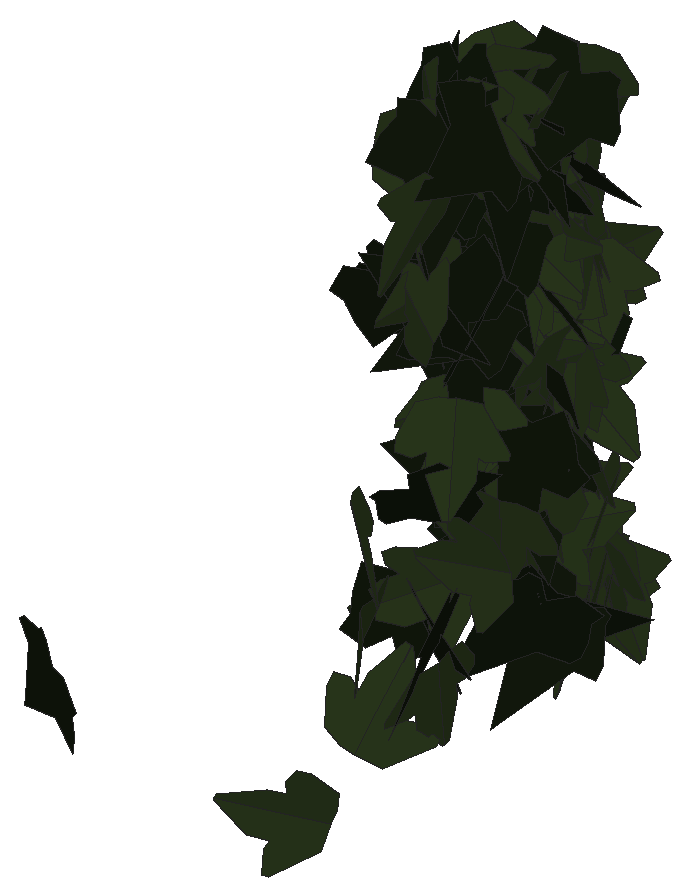
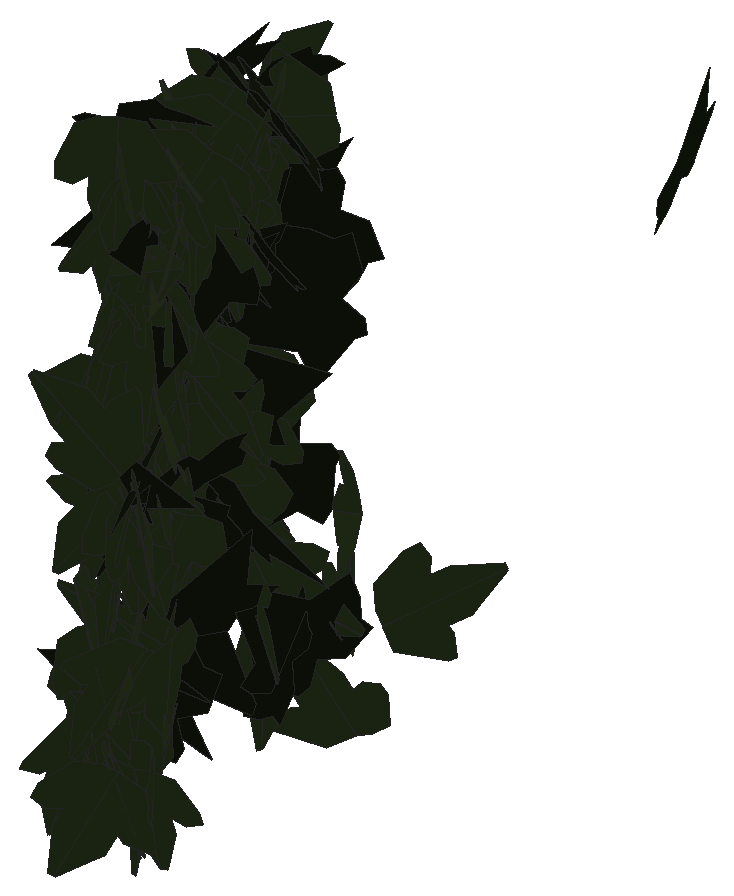
# SketchUp Ruby script. Lengths in inches.
U = 1.inch
M = Sketchup.active_model
def pt(a) = Geom::Point3d.new(a.map { |v| v * U })
def face(e, loops, mat)
  f = e.add_face(loops[0].map { |a| pt(a) })
  loops[1..].each { |l| e.add_face(l.map { |a| pt(a) }).erase! }
  f.material = f.back_material = mat if mat
  f
end
# faces: each face lists its corners as indices into pts; further lists are holes
def faces(e, pts, list, mat = nil) = list.each { |f| face(e, (f[0].is_a?(Array) ? f : [f]).map { |l| l.map { |i| pts[i] } }, mat) }
# xy, xz, yz: faces in a plane at the given z, y or x. An outline is a flat list of corners, or four numbers for a rectangle; further outlines are holes
def ring(l) = l.size == 4 ? [[l[0], l[1]], [l[2], l[1]], [l[2], l[3]], [l[0], l[3]]] : l.each_slice(2).to_a
def flat(e, list, mat, &to3) = list.each { |f| face(e, (f[0].is_a?(Array) ? f : [f]).map { |l| ring(l).map { |u, v| to3.(u, v) } }, mat) }
def xy(e, z, list, mat = nil) = flat(e, list, mat) { |x, y| [x, y, z] }
def xz(e, y, list, mat = nil) = flat(e, list, mat) { |x, z| [x, y, z] }
def yz(e, x, list, mat = nil) = flat(e, list, mat) { |y, z| [x, y, z] }
def lines(e, pts, list) = list.each { |a, b| e.add_line(pt(pts[a]), pt(pts[b])) }
# prism: a flat outline (further loops are holes) pulled along v
def prism(e, loops, v, mat = nil)
  f = face(e, loops, mat); d = Geom::Vector3d.new(v.map { |x| x * U })
  f.pushpull(f.normal.samedirection?(d) ? d.length : -d.length)
end
def box(e, o, s, mat = nil) = prism(e, [[o, [o[0] + s[0], o[1], o[2]], [o[0] + s[0], o[1] + s[1], o[2]], [o[0], o[1] + s[1], o[2]]]], [0, 0, s[2]], mat)
def at(x, y, z, deg = 0) = Geom::Transformation.translation(pt([x, y, z])) * Geom::Transformation.rotation(ORIGIN, Z_AXIS, deg.degrees)
def axes(o, x, y, z) = Geom::Transformation.new([*x, 0, *y, 0, *z, 0, *pt(o).to_a, 1])
def part(name) = M.definitions.add(name)
# library, detail: a bought-in or finely detailed component or shape, given as its bounding box
def library(name, o, s) = part(name).tap { |d| box(d.entities, o, s) }
def detail(e, o, s) = box(e.add_group.entities, o, s)
def put(e, d, t, mat = nil) = e.add_instance(d, t).tap { |i| i.material = mat if mat }
def group(e, t, mat = nil) = e.add_group.tap { |g| g.transformation = t; g.material = mat if mat }.entities
root = M.entities
M.materials.add("efeu1").color = [18, 25, 13]
M.materials.add("efeu2").color = [43, 57, 29]
c1 = part("ivyleaf_9")
p = [[1.54,2.16,1.25],[1.36,2.04,1.19],[-0.21,0.99,0.68],[-0.71,1.11,0.82],[-0.85,0.86,0.67],[-0.8,0.17,0.21],
  [-0.9,-0.01,0.1],[-0.67,-0.16,-0.02],[-0.08,-0.08,-0.05],[-0.03,-0.6,-0.4],[0.65,-0.88,-0.66],[0.83,-0.6,-0.49],
  [1.29,-0.42,-0.43],[1.8125,-0.07,-0.26],[1.21,0.44,0.15]]
faces(c1.entities,p,[[0,1,2,3,4,5,6,7,8,9,10,11,12,13,14]],"efeu1")
c2 = part("ivyleaf_10")
p = [[0,0.5,-0.03],[-0.0625,2.02,-0.43],[-0.19,2.01,-0.46],[-0.54,1.05,-0.29],[-0.52,0.625,-0.18],[-0.83,0.76,-0.28],
  [-1.16,0.64,-0.33],[-1.15,0.33,-0.24],[-0.77,-0.39,0.02],[-0.3,-0.51,0.16],[0.04,-0.48,0.23],[-0.02,2.01,-0.4375],
  [-0.06,2.01,-0.43],[0.04,-0.49,0.23],[0.67,-0.49,0.14],[1.38,0.36,-0.2],[1.375,0.51,-0.24],[0.81,0.65,-0.19],
  [0.62,0.59,-0.15],[0.6,1.09,-0.28],[0.5,1.23,-0.31]]
faces(c2.entities,p,[[0,1,2,3,4,5,6,7,8,9,10],[11,12,0,13,14,15,16,17,18,19,20]],"efeu2")
put(root,c1,axes([54.02,224,209.75],[-0.30675,0.21315,0.33237],[-0.27125,0.19209,-0.37353],[-0.28693,-0.40947,-0.00222]))
put(root,c2,axes([53.75,224.86,213.66],[-0.48275,0.0571,0.117],[-0.11843,-0.00593,-0.48574],[-0.05408,-0.49669,0.01925]))
put(root,c2,axes([53.41,222.89,209.41],[-0.14092,0.21503,-0.42884],[0.24643,-0.35104,-0.257],[-0.4116,-0.28379,-0.00704]))
put(root,c1,axes([53.51,223.33,208.01],[-0.13532,-0.08748,0.47332],[0.40759,0.24072,0.16102],[-0.25605,0.42942,0.00617]))
put(root,c2,axes([53.82,225.09,212.27],[-0.27234,0.3866,0.16238],[-0.24178,0.01341,-0.43745],[-0.3426,-0.31679,0.17964]))
put(root,c1,axes([53.81,223.86,212.63],[-0.44579,0.22427,-0.03121],[-0.02999,0.00983,0.499],[0.22444,0.44677,0.00469]))
put(root,c2,axes([53.75,225.61,207.66],[-0.38667,0.30519,0.08572],[-0.10013,0.01069,-0.48975],[-0.30077,-0.39591,0.05285]))
put(root,c2,axes([53.84,224.62,212.81],[-0.16094,0.39595,0.25946],[-0.25286,0.15977,-0.40067],[-0.4002,-0.26018,0.14881]))
put(root,c1,axes([53.34,223.21,211.88],[0.40872,0.05191,0.28329],[0.27992,0.04414,-0.41194],[-0.06778,0.49533,0.00702]))
put(root,c2,axes([53.54,222.83,208.1875],[0.09583,-0.31513,-0.37618],[0.11096,-0.35945,0.32937],[-0.47802,-0.14661,0.00104]))
put(root,c2,axes([53.75,224.43,213.125],[0.02435,-0.49893,0.02181],[0.00218,-0.02173,-0.49952],[0.4994,0.02442,0.00112]))
put(root,c2,axes([53.54,222.82,207.08],[0.40948,0.1861,-0.21839],[0.19556,0.09746,0.44973],[0.20996,-0.45373,0.00703]))
put(root,c2,axes([54.01,223.42,208.68],[0.21122,0.1027,-0.4414],[-0.4367,-0.08406,-0.22853],[-0.12115,0.48206,0.05419]))
put(root,c2,axes([53.66,223.75,214.1],[-0.18931,0.45646,-0.07616],[0.03121,-0.06951,-0.49416],[-0.46172,-0.19186,-0.00218]))
put(root,c2,axes([53.92,224.33,213.54],[-0.46139,-0.03565,0.18933],[-0.18729,-0.03216,-0.46248],[0.04516,-0.49769,0.01633]))
put(root,c1,axes([53.76,224.69,212.99],[0.24716,0.43383,-0.0265],[-0.0197,-0.01927,-0.49924],[-0.43419,0.24783,0.00757]))
put(root,c2,axes([53.9375,223.74,208.82],[0.21368,-0.25701,-0.37187],[-0.24383,0.28083,-0.33419],[0.38065,0.32416,-0.00531]))
put(root,c2,axes([53.69,225.3125,208.81],[-0.00872,0.49259,-0.08531],[-0.01802,-0.08558,-0.49229],[-0.4996,-0.00551,0.01925]))
put(root,c2,axes([53.82,224.56,212.93],[0.46831,0.06109,0.16419],[-0.16379,-0.0136,0.47222],[0.06216,-0.49607,0.00728]))
put(root,c2,axes([53.74,225.19,213.36],[-0.33463,0.37133,-0.01166],[0.00713,-0.00927,-0.49986],[-0.37144,-0.33471,0.00091]))
put(root,c2,axes([53.83,225.3,212.26],[-0.48587,-0.11751,0.01115],[-0.01089,-0.00242,-0.49988],[0.11753,-0.48599,-0.00021]))
put(root,c2,axes([53.73,225.28,211.49],[0.24357,-0.42005,0.11931],[0.0664,-0.0994,-0.4855],[0.43159,0.25235,0.00736]))
put(root,c2,axes([53.95,224.58,211.49],[0.39899,-0.03659,-0.29912],[-0.29748,0.03146,-0.40065],[0.04814,0.49767,0.00333]))
put(root,c1,axes([53.93,223.26,213.65],[-0.38253,0.28809,-0.14377],[-0.11407,0.08752,0.47888],[0.30109,0.39918,-0.00124]))
put(root,c2,axes([53.55,224.9,214],[0.40968,0.13694,0.25181],[0.23863,0.08039,-0.43196],[-0.15879,0.47412,0.00052]))
put(root,c1,axes([54,224.58,208.78],[-0.3091,-0.37182,0.12732],[0.08841,0.09205,0.48344],[-0.38294,0.32137,0.00884]))
put(root,c1,axes([54.18,223.83,210.89],[-0.052,0.02347,0.49674],[-0.42802,0.25215,-0.05672],[-0.25316,-0.43113,-0.00613]))
put(root,c1,axes([53.61,224.96,210.77],[0.13307,-0.42256,-0.23182],[-0.00313,0.23973,-0.43877],[0.48196,0.11822,0.06115]))
put(root,c2,axes([53.8,224.4,212.92],[-0.0766,0.26517,0.41691],[0.1201,-0.39925,0.276],[0.47928,0.14243,-0.00253]))
put(root,c2,axes([53.86,224.07,210.5],[-0.07448,0.0835,0.48732],[0.03929,-0.49026,0.09001],[0.49286,0.0517,0.06646]))
put(root,c2,axes([53.86,224.87,212.75],[-0.00923,0.02087,0.49948],[0.05468,-0.49652,0.02175],[0.49692,0.05503,0.00688]))
put(root,c2,axes([53.79,225.57,207.49],[0.49967,0.01748,-0.00456],[-0.00396,-0.01697,-0.4997],[-0.01763,0.49941,-0.01682]))
put(root,c2,axes([54.15,224.96,213.37],[0.16187,0.11508,0.45886],[-0.36267,-0.28121,0.19846],[0.30375,-0.39709,-0.00757]))
put(root,c2,axes([53.92,224.78,212.84],[-0.04716,-0.49774,-0.00523],[0.00083,0.00518,-0.49997],[0.49777,-0.04717,0.00034]))
put(root,c2,axes([54.04,224.72,212.47],[0.18178,-0.01875,0.46541],[-0.28193,0.39326,0.12596],[-0.37077,-0.30822,0.1324]))
put(root,c2,axes([53.99,225.39,210.56],[0.25234,-0.39486,-0.17438],[-0.08208,0.15441,-0.46842],[0.42378,0.26503,0.01311]))
put(root,c1,axes([53.57,223.625,208.08],[0.28672,-0.03915,-0.40775],[0.4073,-0.02566,0.28887],[-0.04355,-0.4978,0.01718]))
put(root,c1,axes([53.8,223.97,214.31],[-0.29663,-0.17156,-0.36411],[0.38816,-0.00225,-0.31516],[0.1065,-0.46964,0.13452]))
put(root,c2,axes([53.82,225.17,210.68],[0.15736,-0.35134,0.31906],[0.21658,-0.24594,-0.37763],[0.42229,0.25705,0.07479]))
put(root,c2,axes([54.18,224.66,207.75],[0.06773,-0.07321,0.48995],[-0.36375,0.32835,0.09934],[-0.3363,-0.3699,-0.00878]))
put(root,c2,axes([53.9,226.03,207.56],[-0.41842,-0.17473,-0.2107],[0.22318,0.00507,-0.4474],[0.15849,-0.46845,0.07375]))
put(root,c2,axes([54.35,225.15,212.64],[-0.15877,0.20146,-0.42919],[-0.3877,0.20537,0.23982],[0.27292,0.40895,0.091]))
put(root,c2,axes([53.85,224.96,209.95],[0.30771,0.35999,0.16038],[0.10825,0.11844,-0.47355],[-0.37894,0.32616,-0.00505]))
put(root,c2,axes([53.84,224.375,214.03],[0.28634,0.25248,0.32289],[0.13852,0.3111,-0.3661],[-0.38577,0.29911,0.10821]))
put(root,c2,axes([53.67,225.21,212.41],[0.00674,0.00743,-0.4999],[0.44003,-0.23742,0.00241],[-0.23734,-0.43997,-0.00974]))
put(root,c2,axes([54.11,225.21,210.11],[-0.06911,-0.48998,0.07172],[-0.02056,-0.06952,-0.49472],[0.49477,-0.07133,-0.01054]))
put(root,c2,axes([53.7,223.14,213.72],[0.06244,0.05576,0.49294],[0.39382,0.29656,-0.08343],[-0.30168,0.39868,-0.00689]))
put(root,c1,axes([53.89,224.11,212.39],[0.17289,-0.37771,-0.27829],[-0.10353,0.25856,-0.41525],[0.45759,0.20121,0.0112]))
put(root,c2,axes([54.31,220.92,207.15],[-0.12601,-0.10424,-0.4725],[-0.3794,-0.28174,0.16334],[-0.3003,0.39969,-0.0081]))
put(root,c2,axes([53.92,223.87,210.59],[0.45188,0.19909,0.0785],[0.07066,0.03432,-0.49379],[-0.20201,0.45737,0.00288]))
put(root,c2,axes([54.09,224.65,212.71],[-0.10829,0.45723,0.17092],[-0.11888,0.14511,-0.46348],[-0.47344,-0.14102,0.07729]))
put(root,c2,axes([53.84,224.87,213.52],[0.07046,-0.11382,0.48175],[0.3216,-0.35939,-0.13195],[0.37631,0.32845,0.02256]))
put(root,c2,axes([53.94,225.57,208.7],[0.12616,0.38725,0.29003],[0.05151,0.28728,-0.40598],[-0.48107,0.13232,0.03259]))
put(root,c1,axes([54.45,225.35,210.65],[-0.17829,0.16495,0.43704],[-0.34403,0.27008,-0.24229],[-0.316,-0.3871,0.01719]))
put(root,c2,axes([54.09,225.05,210.73],[-0.4963,0.05862,-0.01568],[0.01717,0.01174,-0.49957],[-0.0582,-0.49641,-0.01367]))
put(root,c2,axes([53.77,224.99,213.25],[0.37175,-0.08988,-0.32206],[0.30856,-0.09333,0.38221],[-0.12882,-0.48292,-0.01393]))
put(root,c2,axes([54.07,225.55,208.35],[-0.28843,0.38362,0.14016],[0.07961,-0.11549,0.47992],[0.40059,0.29916,0.00554]))
put(root,c2,axes([53.88,224.51,211.81],[0.23982,0.35497,0.25784],[0.14541,0.21293,-0.42839],[-0.41394,0.28046,-0.0011]))
put(root,c2,axes([54.14,225.18,210.19],[-0.30041,-0.39948,-0.01307],[0.01491,0.00514,-0.49975],[0.39941,-0.30065,0.00883]))
put(root,c1,axes([53.74,222.72,212.46],[0.00547,0.01691,-0.49968],[0.35971,0.34693,0.01568],[0.34724,-0.35966,-0.00837]))
put(root,c2,axes([53.94,223.99,213.21],[-0.39984,0.19907,-0.22472],[0.20385,-0.09473,-0.44662],[-0.22039,-0.44877,-0.0054]))
put(root,c2,axes([54.14,224.27,212.6],[-0.39273,-0.30685,-0.04003],[0.03257,0.02333,-0.49839],[0.30773,-0.39408,0.00166]))
put(root,c2,axes([53.85,224.5625,213.57],[0.16987,-0.40237,-0.2434],[0.23173,-0.15357,0.41559],[-0.4092,-0.254,0.13431]))
put(root,c2,axes([54.04,225.57,207.53],[0.37785,-0.31204,0.0993],[0.0702,-0.07091,-0.48994],[0.31984,0.38419,-0.00978]))
put(root,c1,axes([54.21,224.375,213.08],[0.31107,0.29418,-0.25825],[-0.2274,-0.13269,-0.42507],[-0.31863,0.3819,0.05124]))
put(root,c1,axes([54.01,223,209.95],[0.35813,0.33476,0.09837],[0.07151,0.06755,-0.49023],[-0.34151,0.3652,0.00051]))
put(root,c2,axes([54.09,225.61,207.57],[0.32033,-0.37439,0.08496],[0.04792,-0.07079,-0.49264],[0.38091,0.32376,-0.00947]))
put(root,c1,axes([54.24,225.27,210.32],[0.09709,-0.44143,0.21381],[-0.01917,0.21437,0.45131],[-0.49011,-0.09583,0.02471]))
put(root,c2,axes([53.91,225.98,211.23],[-0.30568,-0.12733,0.37463],[0.34535,0.14519,0.33114],[-0.19312,0.4612,-0.00082]))
put(root,c1,axes([53.94,217.23,210.39],[0.27981,-0.25614,-0.32573],[0.28398,-0.1677,0.37581],[-0.30177,-0.39531,0.05163]))
put(root,c2,axes([54.07,224.06,214.05],[-0.40989,-0.18288,-0.22034],[0.22212,0.03973,-0.44619],[0.18071,-0.46365,0.04868]))
put(root,c2,axes([54.16,224.6,213.15],[-0.37925,-0.32006,-0.06109],[0.12059,-0.05078,-0.48258],[0.3027,-0.38077,0.1157]))
put(root,c2,axes([54.22,223.11,207.8125],[-0.07957,-0.47726,-0.12607],[0.02894,0.12297,-0.48378],[0.49278,-0.08429,0.00805]))
put(root,c2,axes([53.97,223.67,209.53],[0.21925,0.17836,-0.41245],[0.30019,0.28337,0.28212],[0.33439,-0.37133,0.01717]))
put(root,c2,axes([54.09,225.35,207.53],[-0.14188,-0.39766,0.26784],[0.08066,0.25554,0.42213],[-0.47261,0.16299,-0.00836]))
put(root,c2,axes([54.22,224.47,208.99],[-0.29379,0.39687,0.07862],[-0.05691,0.05567,-0.49362],[-0.40056,-0.29899,0.01246]))
put(root,c2,axes([53.91,224.57,211.13],[-0.07297,-0.0633,-0.49058],[0.46157,0.16958,-0.09053],[0.17785,-0.46609,0.03368]))
put(root,c2,axes([54.33,225.14,209.93],[-0.28915,0.3744,0.16193],[-0.13814,0.09688,-0.47067],[-0.38381,-0.31692,0.04742]))
put(root,c1,axes([54.2,224.8,211.67],[0.42011,-0.00039,-0.27112],[-0.26204,0.12771,-0.40623],[0.06956,0.48342,0.1071]))
put(root,c2,axes([54.38,225.26,214.08],[-0.4795,-0.12747,0.06187],[-0.05938,-0.01743,-0.49615],[0.12865,-0.48316,0.00158]))
put(root,c1,axes([54.19,223.3,213.98],[-0.13129,-0.47962,-0.05224],[0.00856,0.05181,-0.49723],[0.48238,-0.13145,-0.0054]))
put(root,c1,axes([54.45,223.6875,211.98],[-0.2848,-0.27789,0.30277],[-0.22062,-0.2074,-0.39788],[0.34672,-0.36023,-0.00448]))
put(root,c2,axes([54.29,225.13,210.71],[-0.46309,-0.16922,-0.08313],[0.09083,-0.00707,-0.49163],[0.16521,-0.47044,0.03729]))
put(root,c2,axes([54.3,223.1,212.46],[-0.00473,-0.0254,0.49933],[0.08605,-0.49194,-0.02421],[0.49252,0.08571,0.00902]))
put(root,c2,axes([54.37,225,210.93],[-0.02703,-0.49557,-0.06067],[-0.0011,0.06082,-0.49629],[0.49927,-0.02669,-0.00437]))
put(root,c2,axes([54.53,225.31,208.57],[-0.44533,-0.05677,0.22013],[-0.20784,-0.09449,-0.44483],[0.09211,-0.4877,0.06055]))
put(root,c1,axes([53.97,224.71,213.34],[0.45045,-0.06043,0.20843],[0.20664,-0.02721,-0.45449],[0.06627,0.49559,0.00046]))
put(root,c1,axes([54.24,225.05,209.87],[-0.08379,-0.45631,0.18643],[-0.02604,-0.18475,-0.46389],[0.49224,-0.08744,0.0072]))
put(root,c1,axes([54.53,223.16,212.04],[0.0453,0.06437,0.49377],[-0.44525,-0.21675,0.0691],[0.22294,-0.44596,0.03768]))
put(root,c1,axes([54.55,224.0625,212.74],[-0.49841,-0.00389,-0.03963],[0.03961,0.00335,-0.49842],[0.00414,-0.49997,-0.00303]))
put(root,c2,axes([53.99,224.91,212.13],[-0.11146,-0.00213,0.48741],[0.48493,0.04995,0.11111],[-0.04916,0.49749,-0.00907]))
put(root,c1,axes([54.39,223.05,208.67],[-0.26898,0.22213,-0.3582],[0.27247,-0.23256,-0.34882],[-0.32157,-0.38285,0.00406]))
put(root,c2,axes([54.17,224.49,212.33],[0.16434,0.34369,0.32384],[0.14644,0.2889,-0.38091],[-0.44894,0.22004,-0.0057]))
put(root,c2,axes([54.39,225.27,213.3],[0.05835,-0.03033,-0.49566],[0.02223,0.49873,-0.0279],[0.49609,-0.01879,0.05955]))
put(root,c2,axes([54.48,225.17,209.65],[-0.40807,0.25203,0.14126],[-0.13046,0.05738,-0.47926],[-0.25779,-0.428,0.01893]))
put(root,c2,axes([54.37,224.97,213.86],[0.16072,-0.46226,0.10239],[0.0358,-0.09595,-0.4894],[0.47211,0.16464,0.00226]))
put(root,c2,axes([54.44,225.4,211.35],[0.05303,0.49398,-0.05631],[-0.01876,0.05858,0.4962],[0.49683,-0.05051,0.02475]))
put(root,c2,axes([54.45,225.57,207.98],[0.26809,-0.38253,-0.17833],[-0.06068,0.17414,-0.46475],[0.41767,0.27083,0.04695]))
put(root,c2,axes([54.34,225,213.55],[0.45617,-0.20232,0.0312],[0.028,-0.01383,-0.49902],[0.20278,0.45703,-0.00129]))
put(root,c2,axes([54.45,225.27,212.31],[-0.26725,0.39001,0.16269],[-0.09205,0.13415,-0.47279],[-0.41244,-0.28266,0.0001]))
put(root,c1,axes([54.26,224.59,209.91],[-0.22853,-0.33743,-0.28968],[0.21155,0.204,-0.40452],[0.39118,-0.30745,0.04953]))
put(root,c1,axes([54.11,224.54,213.67],[0.17944,-0.44445,0.14235],[0.15536,-0.08692,-0.46723],[0.44007,0.21191,0.10691]))
put(root,c1,axes([54.73,224.11,209.8],[0.08954,-0.00376,0.4919],[-0.43357,0.23558,0.08072],[-0.23237,-0.44101,0.03893]))
put(root,c2,axes([54.11,223.8,213.98],[-0.20183,0.06311,-0.45308],[0.42856,-0.14714,-0.2114],[-0.16001,-0.47367,0.0053]))
put(root,c2,axes([54.57,223.74,209.52],[-0.48169,-0.10721,0.08053],[-0.07966,-0.01273,-0.49345],[0.10786,-0.4882,-0.00482]))
put(root,c1,axes([54.25,224.18,213.38],[0.06927,-0.46409,0.17268],[0.03633,-0.16913,-0.46912],[0.49384,0.07754,0.0103]))
put(root,c2,axes([54.42,225.74,207.86],[0.01412,0.47983,0.13987],[-0.03042,0.1405,-0.47889],[-0.49887,0.00501,0.03316]))
put(root,c2,axes([54.53,225.4,208.39],[-0.4635,0.18037,0.05131],[-0.04576,0.02388,-0.49733],[-0.18186,-0.46572,-0.00563]))
put(root,c1,axes([54.62,223.0625,211.79],[0.0141,0.28332,0.41174],[-0.01705,0.41193,-0.28288],[-0.49951,-0.00606,0.02128]))
put(root,c2,axes([54.77,222.28,212.43],[0.18653,0.02853,0.46303],[-0.45149,0.12584,0.17412],[-0.1066,-0.48306,0.07271]))
put(root,c2,axes([54.27,225.28,210.27],[0.25177,0.29722,0.31348],[0.1969,0.244,-0.38948],[-0.3845,0.31957,0.00582]))
put(root,c2,axes([54.36,225.35,211.6],[0.35899,0.32982,0.11113],[0.07555,0.08199,-0.48741],[-0.33973,0.36674,0.00903]))
put(root,c2,axes([54.12,225.04,208.71],[0.18924,-0.06194,-0.45864],[0.46227,0.00142,0.19055],[-0.0223,-0.49615,0.0578]))
put(root,c2,axes([54.85,223.14,209.26],[0.12403,-0.00528,-0.48434],[-0.46243,0.14747,-0.12003],[0.14412,0.47773,0.0317]))
put(root,c2,axes([54.4,223.11,210.8],[0.48589,0.10907,0.04491],[0.04181,0.01875,-0.4979],[-0.1103,0.4876,0.0091]))
put(root,c2,axes([54.51,222.57,213.61],[0.00706,-0.36249,0.34431],[0.07536,-0.33964,-0.35912],[0.49424,0.05696,0.04984]))
put(root,c1,axes([54.12,224.71,207.76],[0.17853,-0.09185,0.45792],[0.45229,-0.08824,-0.19404],[0.11646,0.4835,0.05158]))
put(root,c1,axes([54.77,224.13,208.4],[0.00192,0.20581,-0.45567],[-0.14746,-0.43518,-0.19718],[-0.47776,0.13514,0.05903]))
put(root,c2,axes([54.58,225.4375,209.12],[0.25249,-0.42735,-0.06014],[-0.03306,0.05032,-0.49636],[0.4303,0.25463,-0.00284]))
put(root,c2,axes([54.875,224.21,209.87],[-0.29233,0.00473,0.40561],[-0.3915,-0.13415,-0.28059],[0.10617,-0.48164,0.08213]))
put(root,c1,axes([54.61,224.875,214.09],[-0.38976,-0.31285,-0.01462],[0.01274,0.00748,-0.49978],[0.31293,-0.38996,0.00214]))
put(root,c1,axes([54.55,223.7,213.93],[-0.17012,-0.29734,0.36421],[-0.10681,-0.35274,-0.33788],[0.45788,-0.19276,0.0565]))
put(root,c2,axes([54.49,225.38,208.16],[0.3107,-0.3728,0.12034],[0.08589,-0.08503,-0.48517],[0.38221,0.32216,0.01121]))
put(root,c2,axes([54.4375,225.01,210.6875],[0.47803,-0.12618,0.07462],[0.08734,0.04071,-0.49063],[0.11774,0.4821,0.06097]))
put(root,c1,axes([54.68,224.7,208.04],[-0.47337,-0.14806,-0.06324],[0.06067,0.01785,-0.49598],[0.14913,-0.47724,0.00106]))
put(root,c2,axes([54.36,225.24,212.37],[0.40945,-0.16567,0.23432],[0.21788,-0.08625,-0.44169],[0.18677,0.46381,0.00156]))
